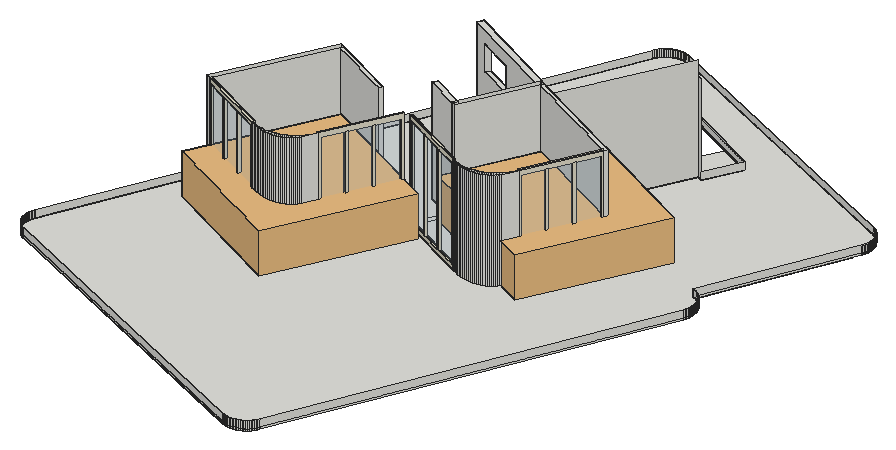
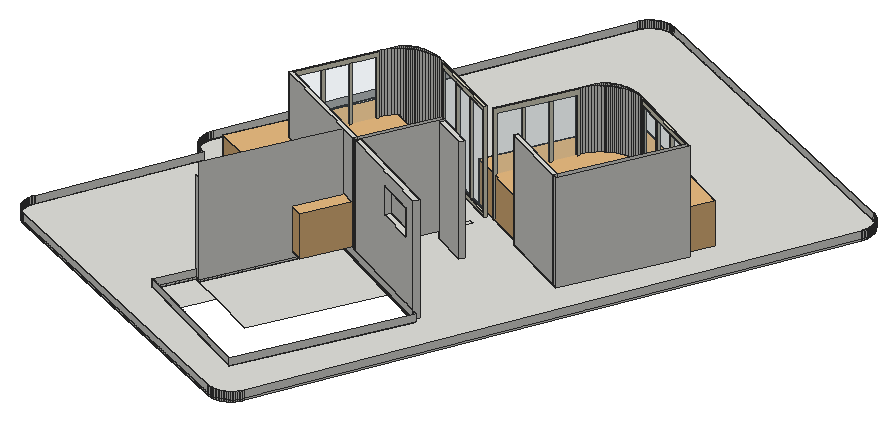
# SketchUp Ruby script. Lengths in inches.
U = 1.inch
M = Sketchup.active_model
def pt(a) = Geom::Point3d.new(a.map { |v| v * U })
def face(e, loops, mat)
  f = e.add_face(loops[0].map { |a| pt(a) })
  loops[1..].each { |l| e.add_face(l.map { |a| pt(a) }).erase! }
  f.material = f.back_material = mat if mat
  f
end
# faces: each face lists its corners as indices into pts; further lists are holes
def faces(e, pts, list, mat = nil) = list.each { |f| face(e, (f[0].is_a?(Array) ? f : [f]).map { |l| l.map { |i| pts[i] } }, mat) }
# xy, xz, yz: faces in a plane at the given z, y or x. An outline is a flat list of corners, or four numbers for a rectangle; further outlines are holes
def ring(l) = l.size == 4 ? [[l[0], l[1]], [l[2], l[1]], [l[2], l[3]], [l[0], l[3]]] : l.each_slice(2).to_a
def flat(e, list, mat, &to3) = list.each { |f| face(e, (f[0].is_a?(Array) ? f : [f]).map { |l| ring(l).map { |u, v| to3.(u, v) } }, mat) }
def xy(e, z, list, mat = nil) = flat(e, list, mat) { |x, y| [x, y, z] }
def xz(e, y, list, mat = nil) = flat(e, list, mat) { |x, z| [x, y, z] }
def yz(e, x, list, mat = nil) = flat(e, list, mat) { |y, z| [x, y, z] }
def lines(e, pts, list) = list.each { |a, b| e.add_line(pt(pts[a]), pt(pts[b])) }
# prism: a flat outline (further loops are holes) pulled along v
def prism(e, loops, v, mat = nil)
  f = face(e, loops, mat); d = Geom::Vector3d.new(v.map { |x| x * U })
  f.pushpull(f.normal.samedirection?(d) ? d.length : -d.length)
end
def box(e, o, s, mat = nil) = prism(e, [[o, [o[0] + s[0], o[1], o[2]], [o[0] + s[0], o[1] + s[1], o[2]], [o[0], o[1] + s[1], o[2]]]], [0, 0, s[2]], mat)
def at(x, y, z, deg = 0) = Geom::Transformation.translation(pt([x, y, z])) * Geom::Transformation.rotation(ORIGIN, Z_AXIS, deg.degrees)
def axes(o, x, y, z) = Geom::Transformation.new([*x, 0, *y, 0, *z, 0, *pt(o).to_a, 1])
def part(name) = M.definitions.add(name)
# library, detail: a bought-in or finely detailed component or shape, given as its bounding box
def library(name, o, s) = part(name).tap { |d| box(d.entities, o, s) }
def detail(e, o, s) = box(e.add_group.entities, o, s)
def put(e, d, t, mat = nil) = e.add_instance(d, t).tap { |i| i.material = mat if mat }
def group(e, t, mat = nil) = e.add_group.tap { |g| g.transformation = t; g.material = mat if mat }.entities
root = M.entities
M.materials.add("Glass").color = [171, 209, 242]
M.materials["Glass"].alpha = 0.09
M.materials.add("Plastic_SSS_01_White").color = [225, 221, 201]
c1 = library("BED_01",[-66.74,-61.37,0],[192.98,188.94,55.24])
c2 = part("Component\#39")
xy(c2.entities,0,[[[104.47,83.98,176.47,131.98],[106.47,85.98,174.47,129.98]],[127.47,85.98,129.47,129.98],[150.47,85.98,152.47,129.98]],"Plastic_SSS_01_White")
xy(c2.entities,2,[[[104.47,83.98,176.47,131.98],[106.47,85.98,174.47,129.98]],[127.47,85.98,129.47,129.98],[150.47,85.98,152.47,129.98]],"Plastic_SSS_01_White")
xz(c2.entities,83.98,[[104.47,0,176.47,2]],"Plastic_SSS_01_White")
xz(c2.entities,85.98,[[106.47,0,127.47,2],[127.47,0,129.47,2],[129.47,0,150.47,2],[150.47,0,152.47,2],[152.47,0,174.47,2]],"Plastic_SSS_01_White")
xz(c2.entities,129.98,[[106.47,0,127.47,2],[127.47,0,129.47,2],[129.47,0,150.47,2],[150.47,0,152.47,2],[152.47,0,174.47,2]],"Plastic_SSS_01_White")
xz(c2.entities,131.98,[[104.47,0,176.47,2]],"Plastic_SSS_01_White")
yz(c2.entities,104.47,[[83.98,0,131.98,2]],"Plastic_SSS_01_White")
yz(c2.entities,106.47,[[85.98,0,129.98,2]],"Plastic_SSS_01_White")
yz(c2.entities,127.47,[[85.98,0,129.98,2]],"Plastic_SSS_01_White")
yz(c2.entities,129.47,[[85.98,0,129.98,2]],"Plastic_SSS_01_White")
yz(c2.entities,150.47,[[85.98,0,129.98,2]],"Plastic_SSS_01_White")
yz(c2.entities,152.47,[[85.98,0,129.98,2]],"Plastic_SSS_01_White")
yz(c2.entities,174.47,[[85.98,0,129.98,2]],"Plastic_SSS_01_White")
yz(c2.entities,176.47,[[83.98,0,131.98,2]],"Plastic_SSS_01_White")
c3 = part("Component\#40")
box(c3.entities,[0,0,0],[67.88,44,0.5])
c4 = part("Component\#43")
put(c4.entities,c2,at(-104.47,-83.98,0))
put(c4.entities,c3,at(2,2,0.7),"Glass")
c5 = part("window")
p = [[-596.28,88.12,20.39],[-668.28,88.12,20.39]]
lines(c5.entities,p,[[0,1]])
put(c5.entities,c4,axes([-668.28,88.12,20.39],[1,0,0],[0,0,1],[0,-1,0]))
xy(root,312.91,[[[841.44,516.19,840.14,516.26,838.84,516.41,837.55,516.64,836.28,516.96,835.03,517.37,833.82,517.85,548.6875,642.03,547.51,642.59,546.36,643.23,545.26,643.94,544.21,644.73,543.22,645.57,542.28,646.49,541.4,647.46,540.59,648.48,539.85,649.56,539.18,650.68,538.58,651.85,538.0625,653.05,537.62,654.28,537.26,655.54,536.99,656.82,536.8,658.12,536.7,659.42,536.68,660.73,536.74,662.04,536.9,663.34,537.13,664.625,537.45,665.89,537.85,667.14,538.34,668.36,741.17,1134.07,741.73,1135.26,742.37,1136.4,743.08,1137.5,743.86,1138.55,744.71,1139.54,745.625,1140.48,746.59,1141.36,747.62,1142.17,748.7,1142.92,749.82,1143.59,750.99,1144.18,752.1875,1144.7,753.42,1145.14,754.68,1145.5,755.96,1145.77,757.26,1145.96,758.56,1146.07,759.87,1146.08,761.18,1146.02,762.48,1145.87,763.76,1145.63,765.03,1145.31,766.28,1144.91,767.49,1144.42,1030.62,1029.82,1031.8,1029.26,1032.95,1028.625,1034.04,1027.91,1035.09,1027.13,1036.09,1026.28,1037.03,1025.37,1037.91,1024.4,1038.72,1023.375,1039.46,1022.3,1040.13,1021.17,1040.73,1020.01,1041.25,1018.81,1041.6875,1017.57,1042.04,1016.31,1042.32,1015.03,1042.51,1013.74,1042.61,1012.44,1042.63,1011.125,1042.57,1009.82,1042.41,1008.52,1042.18,1007.23,1041.86,1005.96,1041.45,1004.72,1040.97,1003.5,985.47,876.0625,989.14,874.47,990.32,873.91,991.46,873.27,992.56,872.56,993.61,871.78,994.61,870.93,995.54,870.01,996.42,869.04,997.23,868.02,997.98,866.94,998.65,865.82,999.24,864.65,999.76,863.45,1000.2,862.22,1000.56,860.96,1000.83,859.68,1001.02,858.38,1001.13,857.08,1001.15,855.77,1001.08,854.46,1000.93,853.16,1000.69,851.875,1000.37,850.61,999.97,849.36,999.49,848.14,860.14,528.2,859.58,527.02,858.94,525.875,858.23,524.78,857.45,523.73,856.6,522.73,855.6875,521.79,854.72,520.91,853.69,520.1,852.61,519.36,851.49,518.6875,850.32,518.09,849.125,517.57,847.89,517.14,846.63,516.78,845.35,516.5,844.06,516.3125,842.75,516.21],[826.625,913.12,877.08,1017.03,881.58,1014.85,897.14,1046.9,866.2,1061.92,780.33,1103.61,714.3125,967.65,757.25,946.81]],[826.625,913.12,877.08,1017.03,850.64,1029.87,807.7,1050.72,757.25,946.81],[881.58,1014.85,897.14,1046.9,866.2,1061.92,850.64,1029.87,877.08,1017.03]])
xy(root,314.6,[[[841.44,516.19,842.75,516.21,844.06,516.3125,845.35,516.5,846.63,516.78,847.89,517.14,849.125,517.57,850.32,518.09,851.49,518.6875,852.61,519.36,853.69,520.1,854.72,520.91,855.6875,521.79,856.6,522.73,857.45,523.73,858.23,524.78,858.94,525.875,859.58,527.02,860.14,528.2,999.49,848.14,999.97,849.36,1000.37,850.61,1000.69,851.875,1000.93,853.16,1001.08,854.46,1001.15,855.77,1001.13,857.08,1001.02,858.38,1000.83,859.68,1000.56,860.96,1000.2,862.22,999.76,863.45,999.24,864.65,998.65,865.82,997.98,866.94,997.23,868.02,996.42,869.04,995.54,870.01,994.61,870.93,993.61,871.78,992.56,872.56,991.46,873.27,990.32,873.91,989.14,874.47,985.47,876.0625,1040.97,1003.5,1041.45,1004.72,1041.86,1005.96,1042.18,1007.23,1042.41,1008.52,1042.57,1009.82,1042.63,1011.125,1042.61,1012.44,1042.51,1013.74,1042.32,1015.03,1042.04,1016.31,1041.6875,1017.57,1041.25,1018.81,1040.73,1020.01,1040.13,1021.17,1039.46,1022.3,1038.72,1023.375,1037.91,1024.4,1037.03,1025.37,1036.09,1026.28,1035.09,1027.13,1034.04,1027.91,1032.95,1028.625,1031.8,1029.26,1030.62,1029.82,767.49,1144.42,766.28,1144.91,765.03,1145.31,763.76,1145.63,762.48,1145.87,761.18,1146.02,759.87,1146.08,758.56,1146.07,757.26,1145.96,755.96,1145.77,754.68,1145.5,753.42,1145.14,752.1875,1144.7,750.99,1144.18,749.82,1143.59,748.7,1142.92,747.62,1142.17,746.59,1141.36,745.625,1140.48,744.71,1139.54,743.86,1138.55,743.08,1137.5,742.37,1136.4,741.73,1135.26,741.17,1134.07,538.34,668.36,537.85,667.14,537.45,665.89,537.13,664.625,536.9,663.34,536.74,662.04,536.68,660.73,536.7,659.42,536.8,658.12,536.99,656.82,537.26,655.54,537.62,654.28,538.0625,653.05,538.58,651.85,539.18,650.68,539.85,649.56,540.59,648.48,541.4,647.46,542.28,646.49,543.22,645.57,544.21,644.73,545.26,643.94,546.36,643.23,547.51,642.59,548.6875,642.03,833.82,517.85,835.03,517.37,836.28,516.96,837.55,516.64,838.84,516.41,840.14,516.26],[826.625,913.12,714.3125,967.65,780.33,1103.61,897.14,1046.9,881.58,1014.85,877.08,1017.03]]])
xy(root,320.68,[[703.25,736.11,701.35,736.17,699.43,736.32,697.49,736.59,695.54,736.95,693.59,737.42,691.66,737.98,689.74,738.64,687.85,739.4,685.99,740.25,681.68,742.34,683.83,741.38,686.04,740.57,688.3,739.9,690.59,739.375,692.92,739.01,695.27,738.79,697.62,738.73,699.98,738.82,702.32,739.06,704.64,739.46,706.02,739.79,706.96,739.93,708.44,740.24,709.88,740.65,711.25,741.13,712.5625,741.7,713.8,742.36,714.96,743.09,716.04,743.89,716.26,744.08,717.58,744.92,719.49,746.3,721.3,747.81,723.01,749.43,724.61,751.16,726.1,752.99,727.46,754.91,728.6875,756.92,729.79,759,723.97,747.02,723.26,745.72,722.43,744.47,721.5,743.3,720.45,742.2,719.29,741.1875,718.04,740.25,716.69,739.4,715.25,738.65,713.73,737.98,712.14,737.42,710.47,736.95,708.74,736.59,706.96,736.32,705.125,736.17],[616.59,773.95,612.69,775.84,618.5,787.81,622.4,785.91],[851.79,784.02,849.89,784.07,847.96,784.23,846.02,784.49,844.07,784.86,842.125,785.32,840.19,785.89,838.27,786.55,836.38,787.31,834.52,788.16,830.21,790.25,832.36,789.29,834.57,788.47,836.83,787.8,839.13,787.28,841.46,786.91,843.8,786.7,846.16,786.63,848.51,786.73,850.85,786.97,853.18,787.37,854.56,787.7,855.49,787.84,856.98,788.15,858.41,788.55,859.79,789.04,861.1,789.61,862.34,790.26,863.5,790.99,864.58,791.8,864.79,791.99,866.12,792.82,868.03,794.21,869.84,795.71,871.55,797.33,873.15,799.0625,874.63,800.89,875.99,802.82,877.22,804.82,878.32,806.91,872.5,794.93,871.79,793.62,870.97,792.38,870.03,791.21,868.98,790.11,867.83,789.09,866.57,788.16,865.23,787.31,863.79,786.55,862.27,785.89,860.67,785.32,859,784.86,857.28,784.49,855.49,784.23,853.66,784.07],[622.4,785.91,618.5,787.81,659.85,872.97,663.75,871.08],[770.93,833.82,767.03,835.71,776.95,856.13,780.85,854.24],
  [780.85,854.24,776.95,856.13,808.39,920.88,812.29,918.98]])
p = [[840.14,516.26,312.91],[841.44,516.19,312.91],[841.44,516.19,314.6],[840.14,516.26,314.6],[842.75,516.21,312.91],[842.75,516.21,314.6],
  [844.06,516.3125,312.91],[844.06,516.3125,314.6],[838.84,516.41,312.91],[838.84,516.41,314.6],[845.35,516.5,312.91],[845.35,516.5,314.6],
  [837.55,516.64,312.91],[837.55,516.64,314.6],[846.63,516.78,312.91],[846.63,516.78,314.6],[836.28,516.96,312.91],[836.28,516.96,314.6],
  [847.89,517.14,312.91],[847.89,517.14,314.6],[835.03,517.37,312.91],[835.03,517.37,314.6],[849.125,517.57,312.91],[849.125,517.57,314.6],
  [833.82,517.85,312.91],[833.82,517.85,314.6],[850.32,518.09,312.91],[850.32,518.09,314.6],[548.6875,642.03,312.91],[548.6875,642.03,314.6],
  [851.49,518.6875,312.91],[851.49,518.6875,314.6],[852.61,519.36,312.91],[852.61,519.36,314.6],[853.69,520.1,312.91],[853.69,520.1,314.6],
  [854.72,520.91,312.91],[854.72,520.91,314.6],[855.6875,521.79,312.91],[855.6875,521.79,314.6],[856.6,522.73,312.91],[856.6,522.73,314.6],
  [857.45,523.73,312.91],[857.45,523.73,314.6],[858.23,524.78,312.91],[858.23,524.78,314.6],[858.94,525.875,312.91],[858.94,525.875,314.6],
  [859.58,527.02,312.91],[859.58,527.02,314.6],[860.14,528.2,312.91],[860.14,528.2,314.6],[999.49,848.14,312.91],[999.49,848.14,314.6],
  [547.51,642.59,312.91],[547.51,642.59,314.6],[546.36,643.23,312.91],[546.36,643.23,314.6],[545.26,643.94,312.91],[545.26,643.94,314.6],
  [544.21,644.73,312.91],[544.21,644.73,314.6],[543.22,645.57,312.91],[543.22,645.57,314.6],[542.28,646.49,312.91],[542.28,646.49,314.6],
  [541.4,647.46,312.91],[541.4,647.46,314.6],[540.59,648.48,312.91],[540.59,648.48,314.6],[539.85,649.56,312.91],[539.85,649.56,314.6],
  [539.18,650.68,312.91],[539.18,650.68,314.6],[538.58,651.85,312.91],[538.58,651.85,314.6],[538.0625,653.05,312.91],[538.0625,653.05,314.6],
  [537.62,654.28,312.91],[537.62,654.28,314.6],[537.26,655.54,312.91],[537.26,655.54,314.6],[536.99,656.82,312.91],[536.99,656.82,314.6],
  [536.8,658.12,312.91],[536.8,658.12,314.6],[536.7,659.42,312.91],[536.7,659.42,314.6],[536.68,660.73,312.91],[536.68,660.73,314.6],
  [536.74,662.04,312.91],[536.74,662.04,314.6],[536.9,663.34,312.91],[536.9,663.34,314.6],[537.13,664.625,312.91],[537.13,664.625,314.6],
  [537.45,665.89,312.91],[537.45,665.89,314.6],[537.85,667.14,312.91],[537.85,667.14,314.6],[538.34,668.36,312.91],[538.34,668.36,314.6],
  [741.17,1134.07,312.91],[741.17,1134.07,314.6],[999.97,849.36,312.91],[999.97,849.36,314.6],[1000.37,850.61,312.91],[1000.37,850.61,314.6],
  [1000.69,851.875,312.91],[1000.69,851.875,314.6],[1000.93,853.16,312.91],[1000.93,853.16,314.6],[1001.08,854.46,312.91],[1001.08,854.46,314.6],
  [1001.15,855.77,312.91],[1001.15,855.77,314.6],[1001.13,857.08,312.91],[1001.13,857.08,314.6],[1001.02,858.38,312.91],[1001.02,858.38,314.6],
  [1000.83,859.68,312.91],[1000.83,859.68,314.6],[1000.56,860.96,312.91],[1000.56,860.96,314.6],[1000.2,862.22,312.91],[1000.2,862.22,314.6],
  [999.76,863.45,312.91],[999.76,863.45,314.6],[999.24,864.65,312.91],[999.24,864.65,314.6],[998.65,865.82,312.91],[998.65,865.82,314.6],
  [997.98,866.94,312.91],[997.98,866.94,314.6],[997.23,868.02,312.91],[997.23,868.02,314.6],[996.42,869.04,312.91],[996.42,869.04,314.6],
  [995.54,870.01,312.91],[995.54,870.01,314.6],[994.61,870.93,312.91],[994.61,870.93,314.6],[993.61,871.78,312.91],[993.61,871.78,314.6],
  [992.56,872.56,312.91],[992.56,872.56,314.6],[991.46,873.27,312.91],[991.46,873.27,314.6],[990.32,873.91,312.91],[990.32,873.91,314.6],
  [989.14,874.47,312.91],[989.14,874.47,314.6],[985.47,876.0625,312.91],[985.47,876.0625,314.6],[1040.97,1003.5,312.91],[1040.97,1003.5,314.6],
  [826.625,913.12,312.91],[757.25,946.81,312.91],[714.3125,967.65,312.91],[714.3125,967.65,314.6],[826.625,913.12,314.6],[877.08,1017.03,314.6],
  [877.08,1017.03,312.91],[780.33,1103.61,312.91],[780.33,1103.61,314.6],[1041.45,1004.72,312.91],[1041.45,1004.72,314.6],[1041.86,1005.96,312.91],
  [1041.86,1005.96,314.6],[1042.18,1007.23,312.91],[1042.18,1007.23,314.6],[1042.41,1008.52,312.91],[1042.41,1008.52,314.6],[1042.57,1009.82,312.91],
  [1042.57,1009.82,314.6],[1042.63,1011.125,312.91],[1042.63,1011.125,314.6],[1042.61,1012.44,312.91],[1042.61,1012.44,314.6],[1042.51,1013.74,312.91],
  [1042.51,1013.74,314.6],[1042.32,1015.03,312.91],[1042.32,1015.03,314.6],[881.58,1014.85,314.6],[881.58,1014.85,312.91],[897.14,1046.9,312.91],
  [897.14,1046.9,314.6],[1042.04,1016.31,312.91],[1042.04,1016.31,314.6],[1041.6875,1017.57,312.91],[1041.6875,1017.57,314.6],[1041.25,1018.81,312.91],
  [1041.25,1018.81,314.6],[1040.73,1020.01,312.91],[1040.73,1020.01,314.6],[1040.13,1021.17,312.91],[1040.13,1021.17,314.6],[1039.46,1022.3,312.91],
  [1039.46,1022.3,314.6],[1038.72,1023.375,312.91],[1038.72,1023.375,314.6],[1037.91,1024.4,312.91],[1037.91,1024.4,314.6],[1037.03,1025.37,312.91],
  [1037.03,1025.37,314.6],[1036.09,1026.28,312.91],[1036.09,1026.28,314.6],[1035.09,1027.13,312.91],[1035.09,1027.13,314.6],[1034.04,1027.91,312.91],
  [1034.04,1027.91,314.6],[1032.95,1028.625,312.91],[1032.95,1028.625,314.6],[1031.8,1029.26,312.91],[1031.8,1029.26,314.6],[1030.62,1029.82,312.91],
  [1030.62,1029.82,314.6],[767.49,1144.42,312.91],[767.49,1144.42,314.6],[866.2,1061.92,312.91],[741.73,1135.26,312.91],[741.73,1135.26,314.6],
  [742.37,1136.4,312.91],[742.37,1136.4,314.6],[743.08,1137.5,312.91],[743.08,1137.5,314.6],[743.86,1138.55,312.91],[743.86,1138.55,314.6],
  [744.71,1139.54,312.91],[744.71,1139.54,314.6],[745.625,1140.48,312.91],[745.625,1140.48,314.6],[746.59,1141.36,312.91],[746.59,1141.36,314.6],
  [747.62,1142.17,312.91],[747.62,1142.17,314.6],[748.7,1142.92,312.91],[748.7,1142.92,314.6],[749.82,1143.59,312.91],[749.82,1143.59,314.6],
  [750.99,1144.18,312.91],[750.99,1144.18,314.6],[752.1875,1144.7,312.91],[752.1875,1144.7,314.6],[766.28,1144.91,312.91],[766.28,1144.91,314.6],
  [753.42,1145.14,312.91],[753.42,1145.14,314.6],[765.03,1145.31,312.91],[765.03,1145.31,314.6],[754.68,1145.5,312.91],[754.68,1145.5,314.6],
  [763.76,1145.63,312.91],[763.76,1145.63,314.6],[755.96,1145.77,312.91],[755.96,1145.77,314.6],[762.48,1145.87,312.91],[762.48,1145.87,314.6],
  [757.26,1145.96,312.91],[757.26,1145.96,314.6],[761.18,1146.02,312.91],[761.18,1146.02,314.6],[758.56,1146.07,312.91],[758.56,1146.07,314.6],
  [759.87,1146.08,312.91],[759.87,1146.08,314.6],[841.44,516.19,321.27],[840.14,516.26,321.27],[842.75,516.21,321.27],[844.06,516.3125,321.27],
  [838.84,516.41,321.27],[845.35,516.5,321.27],[837.55,516.64,321.27],[846.63,516.78,321.27],[836.28,516.96,321.27],[847.89,517.14,321.27],
  [835.03,517.37,321.27],[849.125,517.57,321.27],[833.82,517.85,321.27],[850.32,518.09,321.27],[548.6875,642.03,321.27],[851.49,518.6875,321.27],
  [852.61,519.36,321.27],[853.69,520.1,321.27],[854.72,520.91,321.27],[855.6875,521.79,321.27],[856.6,522.73,321.27],[857.45,523.73,321.27],
  [858.23,524.78,321.27],[858.94,525.875,321.27],[859.58,527.02,321.27],[860.14,528.2,321.27],[999.49,848.14,321.27],[547.51,642.59,321.27],
  [546.36,643.23,321.27],[545.26,643.94,321.27],[544.21,644.73,321.27],[543.22,645.57,321.27],[542.28,646.49,321.27],[541.4,647.46,321.27],
  [540.59,648.48,321.27],[539.85,649.56,321.27],[539.18,650.68,321.27],[538.58,651.85,321.27],[538.0625,653.05,321.27],[537.62,654.28,321.27],
  [537.26,655.54,321.27],[536.99,656.82,321.27],[536.8,658.12,321.27],[536.7,659.42,321.27],[536.68,660.73,321.27],[536.74,662.04,321.27],
  [536.9,663.34,321.27],[537.13,664.625,321.27],[537.45,665.89,321.27],[537.85,667.14,321.27],[538.34,668.36,321.27],[741.17,1134.07,321.27],
  [999.97,849.36,321.27],[1000.37,850.61,321.27],[1000.69,851.875,321.27],[1000.93,853.16,321.27],[1001.08,854.46,321.27],[1001.15,855.77,321.27],
  [1001.13,857.08,321.27],[1001.02,858.38,321.27],[1000.83,859.68,321.27],[1000.56,860.96,321.27],[1000.2,862.22,321.27],[999.76,863.45,321.27],
  [999.24,864.65,321.27],[998.65,865.82,321.27],[997.98,866.94,321.27],[997.23,868.02,321.27],[996.42,869.04,321.27],[995.54,870.01,321.27],
  [994.61,870.93,321.27],[993.61,871.78,321.27],[992.56,872.56,321.27],[991.46,873.27,321.27],[990.32,873.91,321.27],[989.14,874.47,321.27],
  [985.47,876.0625,321.27],[1040.97,1003.5,321.27],[826.625,913.12,321.27],[714.3125,967.65,321.27],[718.8125,965.47,321.27],[728.33,960.84,321.27],
  [729.18,960.43,321.27],[730.32,959.88,321.27],[731.17,959.47,321.27],[826.625,913.12,412.84],[841.08,942.9,412.84],[841.92,944.62,412.84],
  [877.08,1017.03,412.84],[877.08,1017.03,399.22],[780.33,1103.61,321.27],[1041.45,1004.72,321.27],[1041.86,1005.96,321.27],[1042.18,1007.23,321.27],
  [1042.41,1008.52,321.27],[1042.57,1009.82,321.27],[1042.63,1011.125,321.27],[1042.61,1012.44,321.27],[1042.51,1013.74,321.27],[1042.32,1015.03,321.27],
  [881.58,1014.85,321.27],[881.58,1014.85,399.22],[896.8,1046.1875,321.27],[897.14,1046.9,321.27],[1042.04,1016.31,321.27],[1041.6875,1017.57,321.27],
  [1041.25,1018.81,321.27],[1040.73,1020.01,321.27],[1040.13,1021.17,321.27],[1039.46,1022.3,321.27],[1038.72,1023.375,321.27],[1037.91,1024.4,321.27],
  [1037.03,1025.37,321.27],[1036.09,1026.28,321.27],[1035.09,1027.13,321.27],[1034.04,1027.91,321.27],[1032.95,1028.625,321.27],[1031.8,1029.26,321.27],
  [1030.62,1029.82,321.27],[767.49,1144.42,321.27],[784.83,1101.43,321.27],[741.73,1135.26,321.27],[742.37,1136.4,321.27],[743.08,1137.5,321.27],
  [743.86,1138.55,321.27],[744.71,1139.54,321.27],[745.625,1140.48,321.27],[746.59,1141.36,321.27],[747.62,1142.17,321.27],[748.7,1142.92,321.27],
  [749.82,1143.59,321.27],[750.99,1144.18,321.27],[752.1875,1144.7,321.27],[766.28,1144.91,321.27],[753.42,1145.14,321.27],[765.03,1145.31,321.27],
  [754.68,1145.5,321.27],[763.76,1145.63,321.27],[755.96,1145.77,321.27],[762.48,1145.87,321.27],[757.26,1145.96,321.27],[761.18,1146.02,321.27],
  [758.56,1146.07,321.27],[759.87,1146.08,321.27],[701.35,736.17,412.84],[701.35,736.17,320.68],[703.25,736.11,320.68],[703.25,736.11,412.84],
  [705.125,736.17,320.68],[705.125,736.17,412.84],[699.43,736.32,412.84],[699.43,736.32,320.68],[706.96,736.32,320.68],[706.96,736.32,412.84],
  [697.49,736.59,412.84],[697.49,736.59,320.68],[708.74,736.59,320.68],[708.74,736.59,412.84],[695.54,736.95,412.84],[695.54,736.95,320.68],
  [710.47,736.95,320.68],[710.47,736.95,412.84],[693.59,737.42,412.84],[693.59,737.42,320.68],[712.14,737.42,320.68],[712.14,737.42,412.84],
  [691.66,737.98,412.84],[691.66,737.98,320.68],[713.73,737.98,320.68],[713.73,737.98,412.84],[689.74,738.64,412.84],[689.74,738.64,320.68],
  [715.25,738.65,320.68],[715.25,738.65,412.84],[687.85,739.4,412.84],[687.85,739.4,320.68],[716.69,739.4,320.68],[716.69,739.4,412.84],
  [697.62,738.73,412.84],[697.62,738.73,320.68],[695.27,738.79,320.68],[695.27,738.79,412.84],[699.98,738.82,412.84],[699.98,738.82,320.68],
  [692.92,739.01,320.68],[692.92,739.01,412.84],[702.32,739.06,412.84],[702.32,739.06,320.68],[690.59,739.375,320.68],[690.59,739.375,412.84],
  [704.64,739.46,412.84],[704.64,739.46,320.68],[685.99,740.25,412.84],[685.99,740.25,320.68],[688.3,739.9,320.68],[688.3,739.9,412.84],
  [718.04,740.25,320.68],[718.04,740.25,412.84],[706.02,739.79,412.84],[706.02,739.79,320.68],[706.96,739.93,320.68],[706.96,739.93,412.84],
  [686.04,740.57,320.68],[686.04,740.57,412.84],[708.44,740.24,412.84],[708.44,740.24,320.68],[681.68,742.34,412.84],[681.68,742.34,320.68],
  [709.88,740.65,412.84],[709.88,740.65,320.68],[719.29,741.1875,320.68],[719.29,741.1875,412.84],[683.83,741.38,320.68],[683.83,741.38,412.84],
  [711.25,741.13,412.84],[711.25,741.13,320.68],[712.5625,741.7,412.84],[712.5625,741.7,320.68],[720.45,742.2,320.68],[720.45,742.2,412.84],
  [713.8,742.36,412.84],[713.8,742.36,320.68],[721.5,743.3,320.68],[721.5,743.3,412.84],[714.96,743.09,412.84],[714.96,743.09,320.68],
  [716.04,743.89,412.84],[716.04,743.89,320.68],[722.43,744.47,320.68],[722.43,744.47,412.84],[716.26,744.08,412.84],[716.26,744.08,320.68],
  [717.58,744.92,412.84],[717.58,744.92,320.68],[723.26,745.72,320.68],[723.26,745.72,412.84],[719.49,746.3,412.84],[719.49,746.3,320.68],
  [723.97,747.02,320.68],[723.97,747.02,412.84],[721.3,747.81,412.84],[721.3,747.81,320.68],[729.79,759,320.68],[729.79,759,412.84],
  [723.01,749.43,412.84],[723.01,749.43,320.68],[724.61,751.16,412.84],[724.61,751.16,320.68],[726.1,752.99,412.84],[726.1,752.99,320.68],
  [727.46,754.91,412.84],[727.46,754.91,320.68],[728.6875,756.92,412.84],[728.6875,756.92,320.68],[612.69,775.84,412.84],[612.69,775.84,320.68],
  [616.59,773.95,320.68],[616.59,773.95,412.84],[622.4,785.91,320.68],[663.75,871.08,320.68],[663.75,871.08,412.84],[618.5,787.81,320.68],
  [659.85,872.97,412.84],[659.85,872.97,320.68],[849.89,784.07,412.84],[849.89,784.07,320.68],[851.79,784.02,320.68],[851.79,784.02,412.84],
  [853.66,784.07,320.68],[853.66,784.07,412.84],[847.96,784.23,412.84],[847.96,784.23,320.68],[855.49,784.23,320.68],[855.49,784.23,412.84],
  [846.02,784.49,412.84],[846.02,784.49,320.68],[857.28,784.49,320.68],[857.28,784.49,412.84],[844.07,784.86,412.84],[844.07,784.86,320.68],
  [859,784.86,320.68],[859,784.86,412.84],[842.125,785.32,412.84],[842.125,785.32,320.68],[860.67,785.32,320.68],[860.67,785.32,412.84],
  [840.19,785.89,412.84],[840.19,785.89,320.68],[862.27,785.89,320.68],[862.27,785.89,412.84],[838.27,786.55,412.84],[838.27,786.55,320.68],
  [863.79,786.55,320.68],[863.79,786.55,412.84],[836.38,787.31,412.84],[836.38,787.31,320.68],[846.16,786.63,412.84],[846.16,786.63,320.68],
  [843.8,786.7,320.68],[843.8,786.7,412.84],[848.51,786.73,412.84],[848.51,786.73,320.68],[865.23,787.31,320.68],[865.23,787.31,412.84],
  [841.46,786.91,320.68],[841.46,786.91,412.84],[850.85,786.97,412.84],[850.85,786.97,320.68],[839.13,787.28,320.68],[839.13,787.28,412.84],
  [853.18,787.37,412.84],[853.18,787.37,320.68],[834.52,788.16,412.84],[834.52,788.16,320.68],[836.83,787.8,320.68],[836.83,787.8,412.84],
  [866.57,788.16,320.68],[866.57,788.16,412.84],[854.56,787.7,412.84],[854.56,787.7,320.68],[855.49,787.84,320.68],[855.49,787.84,412.84],
  [834.57,788.47,320.68],[834.57,788.47,412.84],[856.98,788.15,412.84],[856.98,788.15,320.68],[830.21,790.25,412.84],[830.21,790.25,320.68],
  [858.41,788.55,412.84],[858.41,788.55,320.68],[867.83,789.09,320.68],[867.83,789.09,412.84],[832.36,789.29,320.68],[832.36,789.29,412.84],
  [859.79,789.04,412.84],[859.79,789.04,320.68],[861.1,789.61,412.84],[861.1,789.61,320.68],[868.98,790.11,320.68],[868.98,790.11,412.84],
  [862.34,790.26,412.84],[862.34,790.26,320.68],[870.03,791.21,320.68],[870.03,791.21,412.84],[863.5,790.99,412.84],[863.5,790.99,320.68],
  [864.58,791.8,412.84],[864.58,791.8,320.68],[870.97,792.38,320.68],[870.97,792.38,412.84],[864.79,791.99,412.84],[864.79,791.99,320.68],
  [866.12,792.82,412.84],[866.12,792.82,320.68],[871.79,793.62,320.68],[871.79,793.62,412.84],[868.03,794.21,412.84],[868.03,794.21,320.68],
  [872.5,794.93,320.68],[872.5,794.93,412.84],[869.84,795.71,412.84],[869.84,795.71,320.68],[878.32,806.91,320.68],[878.32,806.91,412.84],
  [871.55,797.33,412.84],[871.55,797.33,320.68],[873.15,799.0625,412.84],[873.15,799.0625,320.68],[874.63,800.89,412.84],[874.63,800.89,320.68],
  [875.99,802.82,412.84],[875.99,802.82,320.68],[877.22,804.82,412.84],[877.22,804.82,320.68],[776.95,856.13,412.84],[776.95,856.13,320.68],
  [780.85,854.24,320.68],[780.85,854.24,412.84],[812.29,918.98,320.68],[812.29,918.98,412.84],[808.39,920.88,320.68],[808.39,920.88,412.84],
  [984.54,875.2,312],[1037.1,997.48,312],[781.22,1102.31,320.32]]
faces(root,p,[[0,1,2,3],[1,4,5,2],[4,6,7,5],[8,0,3,9],[6,10,11,7],[12,8,9,13],[10,14,15,11],[16,12,13,17],
  [14,18,19,15],[20,16,17,21],[18,22,23,19],[24,20,21,25],[22,26,27,23],[28,24,25,29],[26,30,31,27],[30,32,33,31],
  [32,34,35,33],[34,36,37,35],[36,38,39,37],[38,40,41,39],[40,42,43,41],[42,44,45,43],[44,46,47,45],[46,48,49,47],
  [48,50,51,49],[50,52,53,51],[54,28,29,55],[56,54,55,57],[58,56,57,59],[60,58,59,61],[62,60,61,63],[64,62,63,65],
  [66,64,65,67],[68,66,67,69],[70,68,69,71],[72,70,71,73],[74,72,73,75],[76,74,75,77],[78,76,77,79],[80,78,79,81],
  [82,80,81,83],[84,82,83,85],[86,84,85,87],[88,86,87,89],[90,88,89,91],[92,90,91,93],[94,92,93,95],[96,94,95,97],
  [98,96,97,99],[100,98,99,101],[102,100,101,103],[52,104,105,53],[104,106,107,105],[106,108,109,107],[108,110,111,109],[110,112,113,111],
  [112,114,115,113],[114,116,117,115],[116,118,119,117],[118,120,121,119],[120,122,123,121],[122,124,125,123],[124,126,127,125],[126,128,129,127],
  [128,130,131,129],[130,132,133,131],[132,134,135,133],[134,136,137,135],[136,138,139,137],[138,140,141,139],[140,142,143,141],[142,144,145,143],
  [144,146,147,145],[146,148,149,147],[148,150,151,149],[150,152,153,151],[152,154,155,153],[156,157,158,159,160],[160,161,162,156],[158,163,164,159],
  [154,165,166,155],[165,167,168,166],[167,169,170,168],[169,171,172,170],[171,173,174,172],[173,175,176,174],[175,177,178,176],[177,179,180,178],
  [179,181,182,180],[183,184,162,161],[185,184,183,186],[181,187,188,182],[187,189,190,188],[189,191,192,190],[191,193,194,192],[193,195,196,194],
  [195,197,198,196],[197,199,200,198],[199,201,202,200],[201,203,204,202],[203,205,206,204],[205,207,208,206],[207,209,210,208],[209,211,212,210],
  [211,213,214,212],[213,215,216,214],[215,217,218,216],[164,163,219,185,186],[220,102,103,221],[222,220,221,223],[224,222,223,225],[226,224,225,227],
  [228,226,227,229],[230,228,229,231],[232,230,231,233],[234,232,233,235],[236,234,235,237],[238,236,237,239],[240,238,239,241],[242,240,241,243],
  [217,244,245,218],[246,242,243,247],[244,248,249,245],[250,246,247,251],[248,252,253,249],[254,250,251,255],[252,256,257,253],[258,254,255,259],
  [256,260,261,257],[262,258,259,263],[260,264,265,261],[264,262,263,265],[3,2,266,267],[2,5,268,266],[5,7,269,268],[9,3,267,270],
  [7,11,271,269],[13,9,270,272],[11,15,273,271],[17,13,272,274],[15,19,275,273],[21,17,274,276],[19,23,277,275],[25,21,276,278],
  [23,27,279,277],[29,25,278,280],[27,31,281,279],[31,33,282,281],[33,35,283,282],[35,37,284,283],[37,39,285,284],[39,41,286,285],
  [41,43,287,286],[43,45,288,287],[45,47,289,288],[47,49,290,289],[49,51,291,290],[51,53,292,291],[55,29,280,293],[57,55,293,294],
  [59,57,294,295],[61,59,295,296],[63,61,296,297],[65,63,297,298],[67,65,298,299],[69,67,299,300],[71,69,300,301],[73,71,301,302],
  [75,73,302,303],[77,75,303,304],[79,77,304,305],[81,79,305,306],[83,81,306,307],[85,83,307,308],[87,85,308,309],[89,87,309,310],
  [91,89,310,311],[93,91,311,312],[95,93,312,313],[97,95,313,314],[99,97,314,315],[101,99,315,316],[103,101,316,317],[53,105,318,292],
  [105,107,319,318],[107,109,320,319],[109,111,321,320],[111,113,322,321],[113,115,323,322],[115,117,324,323],[117,119,325,324],[119,121,326,325],
  [121,123,327,326],[123,125,328,327],[125,127,329,328],[127,129,330,329],[129,131,331,330],[131,133,332,331],[133,135,333,332],[135,137,334,333],
  [137,139,335,334],[139,141,336,335],[141,143,337,336],[143,145,338,337],[145,147,339,338],[147,149,340,339],[149,151,341,340],[151,153,342,341],
  [153,155,343,342],[344,160,159,345,346,347,348,349,350],[160,344,351,352,353,354,355,161],[159,164,356,345],[155,166,357,343],[166,168,358,357],[168,170,359,358],[170,172,360,359],
  [172,174,361,360],[174,176,362,361],[176,178,363,362],[178,180,364,363],[180,182,365,364],[366,183,161,355,367],[186,183,366,368,369],[182,188,370,365],
  [188,190,371,370],[190,192,372,371],[192,194,373,372],[194,196,374,373],[196,198,375,374],[198,200,376,375],[200,202,377,376],[202,204,378,377],
  [204,206,379,378],[206,208,380,379],[208,210,381,380],[210,212,382,381],[212,214,383,382],[214,216,384,383],[216,218,385,384],[356,164,186,369,386],
  [221,103,317,387],[223,221,387,388],[225,223,388,389],[227,225,389,390],[229,227,390,391],[231,229,391,392],[233,231,392,393],[235,233,393,394],
  [237,235,394,395],[239,237,395,396],[241,239,396,397],[243,241,397,398],[218,245,399,385],[247,243,398,400],[245,249,401,399],[251,247,400,402],
  [249,253,403,401],[255,251,402,404],[253,257,405,403],[259,255,404,406],[257,261,407,405],[263,259,406,408],[261,265,409,407],[265,263,408,409],
  [410,411,412,413],[413,412,414,415],[416,417,411,410],[415,414,418,419],[420,421,417,416],[419,418,422,423],[424,425,421,420],[423,422,426,427],
  [428,429,425,424],[427,426,430,431],[432,433,429,428],[431,430,434,435],[436,437,433,432],[435,434,438,439],[440,441,437,436],[439,438,442,443],
  [444,445,446,447],[448,449,445,444],[447,446,450,451],[452,453,449,448],[451,450,454,455],[456,457,453,452],[458,459,441,440],[455,454,460,461],
  [443,442,462,463],[457,456,464,465],[466,465,464,467],[461,460,468,469],[467,470,471,466],[458,472,473,459],[470,474,475,471],[463,462,476,477],
  [469,468,478,479],[474,480,481,475],[480,482,483,481],[477,476,484,485],[479,478,473,472],[482,486,487,483],[485,484,488,489],[486,490,491,487],
  [490,492,493,491],[489,488,494,495],[492,496,497,493],[498,499,497,496],[495,494,500,501],[502,503,499,498],[501,500,504,505],[506,507,503,502],
  [504,508,509,505],[510,511,507,506],[512,513,511,510],[514,515,513,512],[516,517,515,514],[518,519,517,516],[509,508,519,518],[520,521,522,523],
  [524,525,526,523,522],[527,521,520,528,529],[530,531,532,533],[533,532,534,535],[536,537,531,530],[535,534,538,539],[540,541,537,536],[539,538,542,543],
  [544,545,541,540],[543,542,546,547],[548,549,545,544],[547,546,550,551],[552,553,549,548],[551,550,554,555],[556,557,553,552],[555,554,558,559],
  [560,561,557,556],[562,563,564,565],[566,567,563,562],[559,558,568,569],[565,564,570,571],[572,573,567,566],[571,570,574,575],[576,577,573,572],
  [578,579,561,560],[575,574,580,581],[569,568,582,583],[577,576,584,585],[586,585,584,587],[581,580,588,589],[587,590,591,586],[578,592,593,579],
  [590,594,595,591],[583,582,596,597],[589,588,598,599],[594,600,601,595],[600,602,603,601],[597,596,604,605],[599,598,593,592],[602,606,607,603],
  [605,604,608,609],[606,610,611,607],[610,612,613,611],[609,608,614,615],[612,616,617,613],[618,619,617,616],[615,614,620,621],[622,623,619,618],
  [621,620,624,625],[626,627,623,622],[624,628,629,625],[630,631,627,626],[632,633,631,630],[634,635,633,632],[636,637,635,634],[638,639,637,636],
  [629,628,639,638],[640,641,642,643],[642,644,645,643],[646,641,640,647],[528,526,525,529],[647,645,644,646]])
lines(root,p,[[648,649],[368,650]])
g1 = group(root,at(616.62,1009.94,312.6,-26.09))
prism(g1,[[[211.4,5,0],[111.34,5,0],[111.34,5,100.23],[211.4,5,100.23]],[[123.95,5,88.23],[123.95,5,64.23],[160.08,5,64.23],[160.08,5,88.23]]],[0,-5,0])
g2 = group(root,at(636.85,924.74,314.79,-26.09))
box(g2,[121.81,0,0],[34.19,5,97.4])
put(root,c1,axes([835,858.15,320.68],[0.61022,-0.2955,0],[0.2955,0.61022,0],[0,0,0.678]))
put(root,c5,axes([1235.87,1346.11,281.52],[0.41911,0.86313,0],[-0.89956,0.4368,0],[0,0,1.92]))
g3 = group(root,at(906.58,869.69,320.68,64.1))
box(g3,[0,-2,0],[3.15,108.36,92.16])
put(root,c5,axes([1087.34,1298.2,281.52],[0.41911,0.86313,0],[-0.89956,0.4368,0],[0,0,1.92]))
put(root,c1,axes([686.47,810.24,320.68],[0.61022,-0.2955,0],[-0.2955,-0.61022,0],[0,0,0.678]))
g4 = group(root,at(758.05,821.79,320.68,64.1))
box(g4,[0,40.33,0],[3.15,66.03,92.16])
put(root,c5,axes([1331.64,451.04,281.52],[0.904,-0.43896,0],[0.4368,0.89956,0],[0,0,1.92]))
put(root,c5,axes([1183.1,403.13,281.52],[0.904,-0.43896,0],[0.4368,0.89956,0],[0,0,1.92]))
